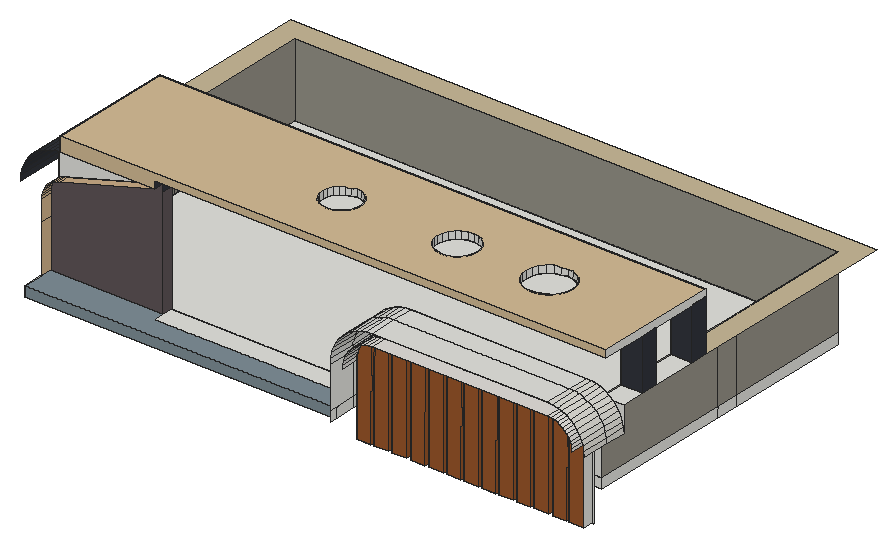
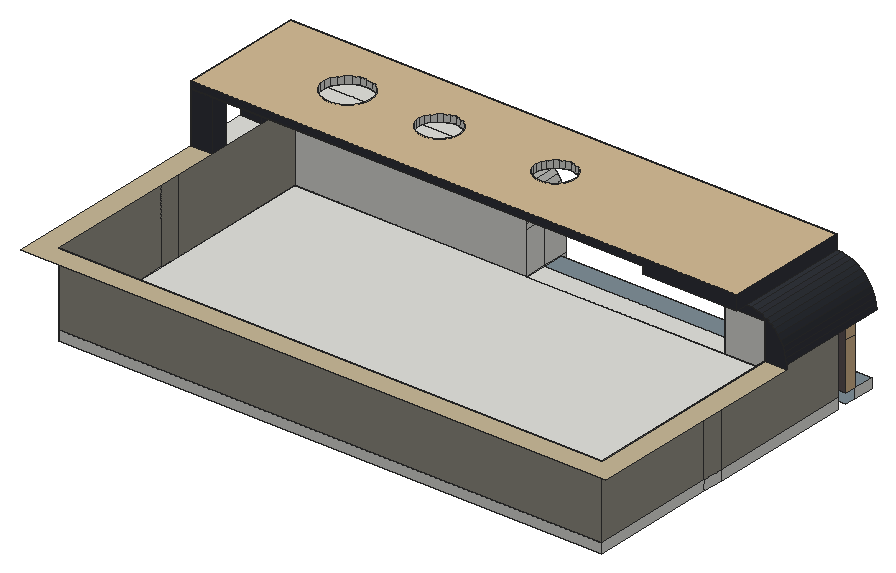
# SketchUp Ruby script. Lengths in inches.
U = 1.inch
M = Sketchup.active_model
def pt(a) = Geom::Point3d.new(a.map { |v| v * U })
def face(e, loops, mat)
  f = e.add_face(loops[0].map { |a| pt(a) })
  loops[1..].each { |l| e.add_face(l.map { |a| pt(a) }).erase! }
  f.material = f.back_material = mat if mat
  f
end
# faces: each face lists its corners as indices into pts; further lists are holes
def faces(e, pts, list, mat = nil) = list.each { |f| face(e, (f[0].is_a?(Array) ? f : [f]).map { |l| l.map { |i| pts[i] } }, mat) }
# xy, xz, yz: faces in a plane at the given z, y or x. An outline is a flat list of corners, or four numbers for a rectangle; further outlines are holes
def ring(l) = l.size == 4 ? [[l[0], l[1]], [l[2], l[1]], [l[2], l[3]], [l[0], l[3]]] : l.each_slice(2).to_a
def flat(e, list, mat, &to3) = list.each { |f| face(e, (f[0].is_a?(Array) ? f : [f]).map { |l| ring(l).map { |u, v| to3.(u, v) } }, mat) }
def xy(e, z, list, mat = nil) = flat(e, list, mat) { |x, y| [x, y, z] }
def xz(e, y, list, mat = nil) = flat(e, list, mat) { |x, z| [x, y, z] }
def yz(e, x, list, mat = nil) = flat(e, list, mat) { |y, z| [x, y, z] }
def lines(e, pts, list) = list.each { |a, b| e.add_line(pt(pts[a]), pt(pts[b])) }
# prism: a flat outline (further loops are holes) pulled along v
def prism(e, loops, v, mat = nil)
  f = face(e, loops, mat); d = Geom::Vector3d.new(v.map { |x| x * U })
  f.pushpull(f.normal.samedirection?(d) ? d.length : -d.length)
end
def box(e, o, s, mat = nil) = prism(e, [[o, [o[0] + s[0], o[1], o[2]], [o[0] + s[0], o[1] + s[1], o[2]], [o[0], o[1] + s[1], o[2]]]], [0, 0, s[2]], mat)
def at(x, y, z, deg = 0) = Geom::Transformation.translation(pt([x, y, z])) * Geom::Transformation.rotation(ORIGIN, Z_AXIS, deg.degrees)
def axes(o, x, y, z) = Geom::Transformation.new([*x, 0, *y, 0, *z, 0, *pt(o).to_a, 1])
def part(name) = M.definitions.add(name)
# library, detail: a bought-in or finely detailed component or shape, given as its bounding box
def library(name, o, s) = part(name).tap { |d| box(d.entities, o, s) }
def detail(e, o, s) = box(e.add_group.entities, o, s)
def put(e, d, t, mat = nil) = e.add_instance(d, t).tap { |i| i.material = mat if mat }
def group(e, t, mat = nil) = e.add_group.tap { |g| g.transformation = t; g.material = mat if mat }.entities
root = M.entities
M.materials.add("[0035_Tan]").color = [210, 180, 140]
M.materials.add("[Asphalt New]").color = [94, 84, 87]
M.materials.add("[Formica Beige]").color = [211, 187, 149]
M.materials.add("[Formica Graystone]1").color = [149, 146, 135]
M.materials.add("[Formica Laminate Dark]").color = [50, 53, 60]
M.materials.add("[Formica Speckled Grey]").color = [127, 142, 150]
M.materials.add("[Quartz Light Brown]").color = [199, 184, 152]
M.materials.add("[Terrazzo Tile Accent]").color = [224, 221, 217]
M.materials.add("[Terrazzo Tile Light]").color = [219, 217, 210]
M.materials.add("[Wood Cherry Original]").color = [152, 86, 42]
xy(root,464.44,[[288.19,14.3125,300.39,22.75],[302.75,14.3125,314.95,22.75],[317.69,14.3125,329.89,22.75],[333.44,14.3125,345.64,22.75],[348.57,14.3125,360.76,22.75],
  [363.5,14.3125,375.7,22.75],[378.19,14.3125,390.39,22.75],[392.75,14.3125,404.95,22.75],[407.44,14.3125,419.64,22.75],[421.94,14.3125,434.14,22.75],
  [436.57,14.3125,448.76,22.75],[452.2,14.3125,464.4,22.75],[466.08,14.3125,478.27,22.75]])
xy(root,479.875,[[112.18,22.75,277.85,40.6875],[17.9375,40.6875,472.4375,162.27],[17.9375,162.27,472.4375,180.28],[17.9375,180.28,472.4375,287.24]])
xy(root,479.875,[[17.9375,5.1875,17.9375,31.75,112.18,31.75,112.18,22.75,277.85,22.75,277.85,5.1875]],"[Formica Speckled Grey]")
xy(root,488.3125,[[112.18,22.75,277.85,40.6875],[17.9375,40.6875,472.4375,287.24]])
xy(root,488.3125,[[17.9375,5.1875,277.85,5.1875,277.85,22.75,112.18,22.75,112.18,31.75,17.9375,31.75]],"[Formica Speckled Grey]")
xy(root,547.97,[[312.85,14.3125,315.18,22.75],[317.69,14.3125,330.02,22.75],[333.44,14.3125,345.77,22.75],[348.57,14.3125,360.9,22.75],[363.5,14.3125,375.83,22.75],
  [378.19,14.3125,390.52,22.75],[392.75,14.3125,405.08,22.75],[407.44,14.3125,419.77,22.75],[421.94,14.3125,434.27,22.75],[436.57,14.3125,448.9,22.75],
  [452.2,14.3125,459.94,22.75]])
xy(root,547.97,[[312.85,0,312.85,14.3125,315.18,14.3125,315.18,22.75,317.69,22.75,317.69,14.3125,330.02,14.3125,330.02,22.75,333.44,22.75,333.44,14.3125,345.77,14.3125,345.77,22.75,348.57,22.75,348.57,14.3125,360.9,14.3125,360.9,22.75,363.5,22.75,363.5,14.3125,375.83,14.3125,375.83,22.75,378.19,22.75,378.19,14.3125,390.52,14.3125,390.52,22.75,392.75,22.75,392.75,14.3125,405.08,14.3125,405.08,22.75,407.44,22.75,407.44,14.3125,419.77,14.3125,419.77,22.75,421.94,22.75,421.94,14.3125,434.27,14.3125,434.27,22.75,436.57,22.75,436.57,14.3125,448.9,14.3125,448.9,22.75,452.2,22.75,452.2,14.3125,459.94,14.3125,459.94,0]],"[Terrazzo Tile Accent]")
xy(root,549.4375,[[472.4375,40.6875,490.375,60.43],[472.4375,60.43,490.375,74.53],[472.4375,74.53,490.375,112.49],[472.4375,112.49,490.375,126.6]])
xy(root,549.4375,[[0,116.75,17.9375,116.75,17.9375,287.24,472.4375,287.24,472.4375,126.6,490.375,126.6,490.375,305.18,0,305.18]],"[Quartz Light Brown]")
xy(root,558.3125,[[312.85,0,459.94,22.75],[312.85,22.75,459.94,40.6875]])
xy(root,579.75,[[17.9375,40.6875,112.18,116.75]])
xy(root,586.1875,[[33.45,22.75,112.18,116.75],[33.45,116.75,112.18,126.6]])
xy(root,592.16,[[[112.18,22.75,490.375,126.6],[402.66,53.0625,407.72,53.73,412.44,55.69,416.49,58.79,419.6,62.85,421.56,67.5625,422.22,72.625,421.56,77.69,419.6,82.41,416.49,86.46,412.44,89.57,407.72,91.52,402.66,92.1875,397.6,91.52,392.88,89.57,388.83,86.46,385.72,82.41,383.76,77.69,383.1,72.625,383.76,67.5625,385.72,62.85,388.83,58.79,392.88,55.69,397.6,53.73],[325.73,55.6875,330.11,56.27,334.2,57.96,337.7,60.65,340.4,64.16,342.09,68.24,342.66,72.625,342.09,77.01,340.4,81.1,337.7,84.6,334.2,87.3,330.11,88.99,325.73,89.5625,321.34,88.99,317.26,87.3,313.75,84.6,311.06,81.1,309.37,77.01,308.79,72.625,309.37,68.24,311.06,64.16,313.75,60.65,317.26,57.96,321.34,56.27],[228.82,56.6875,232.95,57.23,236.79,58.82,240.09,61.36,242.625,64.66,244.22,68.5,244.76,72.625,244.22,76.75,242.625,80.6,240.09,83.9,236.79,86.43,232.95,88.02,228.82,88.5625,224.7,88.02,220.85,86.43,217.55,83.9,215.02,80.6,213.43,76.75,212.89,72.625,213.43,68.5,215.02,64.66,217.55,61.36,220.85,58.82,224.7,57.23]]],"[Formica Beige]")
xy(root,592.3125,[[472.4375,60.43,490.375,74.53],[472.4375,112.49,490.375,126.6]])
xy(root,598.125,[[[33.45,22.75,490.375,126.6],[402.66,53.0625,397.6,53.73,392.88,55.69,388.83,58.79,385.72,62.85,383.76,67.5625,383.1,72.625,383.76,77.69,385.72,82.41,388.83,86.46,392.88,89.57,397.6,91.52,402.66,92.1875,407.72,91.52,412.44,89.57,416.49,86.46,419.6,82.41,421.56,77.69,422.22,72.625,421.56,67.5625,419.6,62.85,416.49,58.79,412.44,55.69,407.72,53.73],[325.73,55.6875,321.34,56.27,317.26,57.96,313.75,60.65,311.06,64.16,309.37,68.24,308.79,72.625,309.37,77.01,311.06,81.1,313.75,84.6,317.26,87.3,321.34,88.99,325.73,89.5625,330.11,88.99,334.2,87.3,337.7,84.6,340.4,81.1,342.09,77.01,342.66,72.625,342.09,68.24,340.4,64.16,337.7,60.65,334.2,57.96,330.11,56.27],[228.82,56.6875,224.7,57.23,220.85,58.82,217.55,61.36,215.02,64.66,213.43,68.5,212.89,72.625,213.43,76.75,215.02,80.6,217.55,83.9,220.85,86.43,224.7,88.02,228.82,88.5625,232.95,88.02,236.79,86.43,240.09,83.9,242.625,80.6,244.22,76.75,244.76,72.625,244.22,68.5,242.625,64.66,240.09,61.36,236.79,58.82,232.95,57.23]]],"[Formica Beige]")
xz(root,5.1875,[[17.9375,479.875,277.85,488.3125]],"[Formica Speckled Grey]")
xz(root,14.3125,[[288.19,464.44,300.39,464.44,300.52,544.67,297.84,542.875,295.41,540.75,293.29,538.32,291.49,535.64,290.07,532.75,289.03,529.69,288.4,526.53,288.19,523.3125],[302.75,464.44,314.95,464.44,315.08,544.67,315.18,547.97,312.85,547.97,309.63,547.76,306.47,547.13,303.41,546.09,302.75,523.3125],[317.69,464.44,329.89,464.44,330.02,544.67,330.02,547.97,317.69,547.97],[333.44,464.44,345.64,464.44,345.77,544.67,345.77,547.97,333.44,547.97],[348.57,464.44,360.76,464.44,360.9,544.67,360.9,547.97,348.57,547.97],
  [363.5,464.44,375.7,464.44,375.83,544.67,375.83,547.97,363.5,547.97],[378.19,464.44,390.39,464.44,390.52,544.67,390.52,547.97,378.19,547.97],[392.75,464.44,404.95,464.44,405.08,544.67,405.08,547.97,392.75,547.97],[407.44,464.44,419.64,464.44,419.77,544.67,419.77,547.97,407.44,547.97],[421.94,464.44,434.14,464.44,434.27,544.67,434.27,547.97,421.94,547.97],
  [436.57,464.44,448.76,464.44,448.9,544.67,448.9,547.97,436.57,547.97],[452.2,464.44,464.4,464.44,464.53,544.67,464.53,547.41,462.57,547.8,459.94,547.97,452.2,547.97],[466.08,464.44,478.27,464.44,478.39,535.8,477.34,537.93,475.88,540.11,474.15,542.09,472.18,543.82,469.99,545.28,467.63,546.44,466.08,546.97]],"[Wood Cherry Original]")
xz(root,22.75,[[288.19,464.44,288.19,523.3125,288.4,526.53,289.03,529.69,290.07,532.75,291.49,535.64,293.29,538.32,295.41,540.75,297.84,542.875,300.52,544.67,300.39,464.44],[302.75,464.44,302.75,523.3125,303.41,546.09,306.47,547.13,309.63,547.76,312.85,547.97,315.18,547.97,315.08,544.67,314.95,464.44],[317.69,464.44,317.69,547.97,330.02,547.97,330.02,544.67,329.89,464.44],[333.44,464.44,333.44,547.97,345.77,547.97,345.77,544.67,345.64,464.44],[348.57,464.44,348.57,547.97,360.9,547.97,360.9,544.67,360.76,464.44],
  [363.5,464.44,363.5,547.97,375.83,547.97,375.83,544.67,375.7,464.44],[378.19,464.44,378.19,547.97,390.52,547.97,390.52,544.67,390.39,464.44],[392.75,464.44,392.75,547.97,405.08,547.97,405.08,544.67,404.95,464.44],[407.44,464.44,407.44,547.97,419.77,547.97,419.77,544.67,419.64,464.44],[421.94,464.44,421.94,547.97,434.27,547.97,434.27,544.67,434.14,464.44],
  [436.57,464.44,436.57,547.97,448.9,547.97,448.9,544.67,448.76,464.44],[452.2,464.44,452.2,547.97,459.94,547.97,462.57,547.8,464.53,547.41,464.53,544.67,464.4,464.44],[466.08,464.44,466.08,546.97,467.63,546.44,469.99,545.28,472.18,543.82,474.15,542.09,475.88,540.11,477.34,537.93,478.39,535.8,478.27,464.44],[478.27,464.44,480.04,464.44,480.04,527.88,479.86,530.5,479.35,533.08,478.51,535.57,478.39,535.8],[478.39,535.8,478.41,544.67,478.41,547.41,476.44,547.8,473.82,547.97,466.08,547.97,466.08,546.97,467.63,546.44,469.99,545.28,472.18,543.82,474.15,542.09,475.88,540.11,477.34,537.93],
  [464.53,547.41,464.53,547.97,459.94,547.97,462.57,547.8]])
xz(root,22.75,[[33.45,586.1875,112.18,586.1875,112.18,592.16,490.375,592.16,490.375,598.125,33.45,598.125]],"[Formica Beige]")
xz(root,22.75,[[300.39,464.44,302.75,464.44,302.75,523.3125,303.41,546.09,300.52,544.67],[314.95,464.44,317.69,464.44,317.69,547.97,315.18,547.97,315.08,544.67],[329.89,464.44,333.44,464.44,333.44,547.97,330.02,547.97,330.02,544.67],[345.64,464.44,348.57,464.44,348.57,547.97,345.77,547.97,345.77,544.67],[360.76,464.44,363.5,464.44,363.5,547.97,360.9,547.97,360.9,544.67],
  [375.7,464.44,378.19,464.44,378.19,547.97,375.83,547.97,375.83,544.67],[390.39,464.44,392.75,464.44,392.75,547.97,390.52,547.97,390.52,544.67],[404.95,464.44,407.44,464.44,407.44,547.97,405.08,547.97,405.08,544.67],[419.64,464.44,421.94,464.44,421.94,547.97,419.77,547.97,419.77,544.67],[434.14,464.44,436.57,464.44,436.57,547.97,434.27,547.97,434.27,544.67],
  [448.76,464.44,452.2,464.44,452.2,547.97,448.9,547.97,448.9,544.67],[464.4,464.44,466.08,464.44,466.08,546.97,465.14,547.29,464.53,547.41,464.53,544.67]],"[Formica Laminate Dark]")
xz(root,31.75,[[17.9375,488.3125,112.18,488.3125,112.18,586.1875,33.29,563.41,31.02,562.96,28.84,562.21,26.77,561.19,24.85,559.91,23.11,558.39,21.59,556.65,20.3,554.73,19.28,552.66,18.54,550.47,18.09,548.21,17.9375,545.9]],"[Asphalt New]")
xz(root,40.6875,[[17.9375,479.875,277.85,488.3125],[277.85,479.875,472.4375,488.3125],[17.9375,488.3125,112.18,579.75],[277.85,488.3125,277.85,523.3125,278.15,527.88,279.04,532.37,280.51,536.71,282.54,540.8125,285.08,544.62,288.1,548.0625,291.54,551.08,295.35,553.625,299.46,555.65,303.79,557.12,308.28,558.01,312.85,558.3125,459.94,558.3125,463.92,558.05,467.82,557.28,471.59,556,472.4375,555.58,472.4375,488.3125],[490.375,527.88,490.375,549.4375,481.42,549.4375,481.46,549.4,484.09,546.41,486.3,543.1,488.06,539.53,489.34,535.76,490.12,531.85],
  [472.4375,549.4375,472.4375,555.58,475.16,554.24,478.47,552.02,481.42,549.4375]])
xz(root,60.43,[[472.4375,549.4375,490.375,592.3125]],"[Formica Laminate Dark]")
xz(root,74.53,[[472.4375,549.4375,490.375,592.3125]],"[Formica Laminate Dark]")
xz(root,112.49,[[472.4375,549.4375,490.375,592.3125]],"[Formica Laminate Dark]")
xz(root,116.75,[[0,549.4375,0,552.73,0.29,557.1,1.14,561.39,2.55,565.54,4.48,569.46,6.91,573.1,9.8,576.39,13.09,579.27,16.73,581.71,17.9375,582.3,17.9375,549.4375],[17.9375,579.75,17.9375,582.3,20.65,583.64,24.8,585.05,29.09,585.9,33.45,586.1875,112.18,586.1875,112.18,579.75]],"[Formica Laminate Dark]")
xz(root,126.6,[[472.4375,592.16,490.375,592.3125]])
xz(root,126.6,[[472.4375,549.4375,490.375,592.16],[33.45,586.1875,33.45,598.125,490.375,598.125,490.375,592.3125,472.4375,592.3125,472.4375,592.16,112.18,592.16,112.18,586.1875]],"[Formica Laminate Dark]")
xz(root,287.24,[[17.9375,479.875,472.4375,488.3125]])
xz(root,287.24,[[17.9375,488.3125,472.4375,549.4375]],"[Formica Graystone]1")
yz(root,17.9375,[[5.1875,479.875,22.75,488.3125],[40.6875,479.875,162.27,488.3125],[162.27,479.875,180.28,488.3125],[180.28,479.875,287.24,488.3125]])
yz(root,17.9375,[[22.75,488.3125,31.75,528.24],[22.75,528.24,31.75,545.9]],"[0035_Tan]")
yz(root,17.9375,[[40.6875,488.3125,162.27,549.4375],[162.27,488.3125,180.28,549.4375],[180.28,488.3125,287.24,549.4375]],"[Formica Graystone]1")
yz(root,17.9375,[[40.6875,549.4375,116.75,579.75]],"[Formica Laminate Dark]")
yz(root,33.45,[[22.75,586.1875,126.6,598.125]],"[Formica Laminate Dark]")
yz(root,112.18,[[31.75,488.3125,40.6875,579.75]],"[Asphalt New]")
yz(root,112.18,[[31.75,579.75,116.75,586.1875],[22.75,586.1875,126.6,592.16]],"[Formica Laminate Dark]")
yz(root,277.85,[[0,479.875,5.1875,488.3125],[5.1875,479.875,22.75,488.3125],[22.75,479.875,40.6875,488.3125],[0,488.3125,22.75,523.3125],[22.75,488.3125,40.6875,523.3125]])
yz(root,288.19,[[14.3125,464.44,22.75,523.3125]])
yz(root,302.75,[[14.3125,464.44,22.75,523.3125]],"[Wood Cherry Original]")
yz(root,317.69,[[14.3125,464.44,22.75,547.97]],"[Wood Cherry Original]")
yz(root,330.02,[[14.3125,544.67,22.75,547.97]],"[Wood Cherry Original]")
yz(root,333.44,[[14.3125,464.44,22.75,547.97]],"[Wood Cherry Original]")
yz(root,345.77,[[14.3125,544.67,22.75,547.97]],"[Wood Cherry Original]")
yz(root,348.57,[[14.3125,464.44,22.75,547.97]],"[Wood Cherry Original]")
yz(root,360.9,[[14.3125,544.67,22.75,547.97]],"[Wood Cherry Original]")
yz(root,363.5,[[14.3125,464.44,22.75,547.97]],"[Wood Cherry Original]")
yz(root,375.83,[[14.3125,544.67,22.75,547.97]],"[Wood Cherry Original]")
yz(root,378.19,[[14.3125,464.44,22.75,547.97]],"[Wood Cherry Original]")
yz(root,390.52,[[14.3125,544.67,22.75,547.97]],"[Wood Cherry Original]")
yz(root,392.75,[[14.3125,464.44,22.75,547.97]],"[Wood Cherry Original]")
yz(root,405.08,[[14.3125,544.67,22.75,547.97]],"[Wood Cherry Original]")
yz(root,407.44,[[14.3125,464.44,22.75,547.97]],"[Wood Cherry Original]")
yz(root,419.77,[[14.3125,544.67,22.75,547.97]],"[Wood Cherry Original]")
yz(root,421.94,[[14.3125,464.44,22.75,547.97]],"[Wood Cherry Original]")
yz(root,434.27,[[14.3125,544.67,22.75,547.97]],"[Wood Cherry Original]")
yz(root,436.57,[[14.3125,464.44,22.75,547.97]],"[Wood Cherry Original]")
yz(root,448.9,[[14.3125,544.67,22.75,547.97]],"[Wood Cherry Original]")
yz(root,452.2,[[14.3125,464.44,22.75,547.97]],"[Wood Cherry Original]")
yz(root,464.53,[[14.3125,544.67,22.75,547.41]],"[Wood Cherry Original]")
yz(root,466.08,[[14.3125,464.44,22.75,546.97]],"[Wood Cherry Original]")
yz(root,472.4375,[[40.6875,479.875,162.27,488.3125],[162.27,479.875,180.28,488.3125],[180.28,479.875,287.24,488.3125]])
yz(root,472.4375,[[40.6875,488.3125,162.27,549.4375],[162.27,488.3125,180.28,549.4375],[180.28,488.3125,287.24,549.4375]],"[Formica Graystone]1")
yz(root,472.4375,[[60.43,549.4375,74.53,592.3125],[112.49,549.4375,126.6,592.3125]],"[Formica Laminate Dark]")
yz(root,490.375,[[22.75,592.16,60.43,592.16,60.43,592.3125,74.53,592.3125,74.53,592.16,112.49,592.16,112.49,592.3125,126.6,592.3125,126.6,598.125,22.75,598.125],[60.43,592.16,74.53,592.3125],[112.49,592.16,126.6,592.3125]])
yz(root,490.375,[[60.43,549.4375,74.53,592.16],[112.49,549.4375,126.6,592.16]],"[Formica Laminate Dark]")
p = [[300.39,22.75,464.44],[300.52,22.75,544.67],[300.52,14.3125,544.67],[300.39,14.3125,464.44],[314.95,22.75,464.44],[315.08,22.75,544.67],
  [315.08,14.3125,544.67],[314.95,14.3125,464.44],[329.89,22.75,464.44],[330.02,22.75,544.67],[330.02,14.3125,544.67],[329.89,14.3125,464.44],
  [345.64,22.75,464.44],[345.77,22.75,544.67],[345.77,14.3125,544.67],[345.64,14.3125,464.44],[360.76,22.75,464.44],[360.9,22.75,544.67],
  [360.9,14.3125,544.67],[360.76,14.3125,464.44],[375.7,22.75,464.44],[375.83,22.75,544.67],[375.83,14.3125,544.67],[375.7,14.3125,464.44],
  [390.39,22.75,464.44],[390.52,22.75,544.67],[390.52,14.3125,544.67],[390.39,14.3125,464.44],[404.95,22.75,464.44],[405.08,22.75,544.67],
  [405.08,14.3125,544.67],[404.95,14.3125,464.44],[419.64,22.75,464.44],[419.77,22.75,544.67],[419.77,14.3125,544.67],[419.64,14.3125,464.44],
  [434.14,22.75,464.44],[434.27,22.75,544.67],[434.27,14.3125,544.67],[434.14,14.3125,464.44],[448.76,22.75,464.44],[448.9,22.75,544.67],
  [448.9,14.3125,544.67],[448.76,14.3125,464.44],[464.4,22.75,464.44],[464.53,22.75,544.67],[464.53,14.3125,544.67],[464.4,14.3125,464.44],
  [478.27,22.75,464.44],[478.39,22.75,535.8],[478.39,14.3125,535.8],[478.27,14.3125,464.44],[278.15,22.75,527.88],[277.85,22.75,523.3125],
  [277.85,0,523.3125],[278.15,0,527.88],[288.19,0,523.3125],[288.19,14.3125,523.3125],[288.4,14.3125,526.53],[288.4,0,526.53],
  [288.19,22.75,523.3125],[288.4,22.75,526.53],[303.41,22.75,546.09],[302.75,22.75,523.3125],[302.75,14.3125,523.3125],[303.41,14.3125,546.09],
  [278.15,40.6875,527.88],[277.85,40.6875,523.3125],[289.03,14.3125,529.69],[289.03,0,529.69],[289.03,22.75,529.69],[279.04,22.75,532.37],
  [279.04,0,532.37],[479.86,22.75,530.5],[480.04,22.75,527.88],[480.04,0,527.88],[479.86,0,530.5],[490.375,22.75,527.88],
  [490.12,22.75,531.85],[490.12,0,531.85],[490.375,0,527.88],[279.04,40.6875,532.37],[490.375,40.6875,527.88],[490.12,40.6875,531.85],
  [290.07,14.3125,532.75],[290.07,0,532.75],[290.07,22.75,532.75],[479.35,22.75,533.08],[479.35,0,533.08],[489.34,22.75,535.76],
  [489.34,0,535.76],[489.34,40.6875,535.76],[280.51,22.75,536.71],[280.51,0,536.71],[280.51,40.6875,536.71],[291.49,14.3125,535.64],
  [291.49,0,535.64],[291.49,22.75,535.64],[478.51,22.75,535.57],[478.51,0,535.57],[293.29,14.3125,538.32],[293.29,0,538.32],
  [477.34,0,537.93],[477.34,14.3125,537.93],[293.29,22.75,538.32],[488.06,22.75,539.53],[488.06,0,539.53],[477.34,22.75,537.93],
  [488.06,40.6875,539.53],[282.54,22.75,540.8125],[282.54,0,540.8125],[282.54,40.6875,540.8125],[475.88,0,540.11],[475.88,14.3125,540.11],
  [475.88,22.75,540.11],[295.41,14.3125,540.75],[295.41,0,540.75],[295.41,22.75,540.75],[486.3,22.75,543.1],[486.3,0,543.1],
  [486.3,40.6875,543.1],[474.15,0,542.09],[474.15,14.3125,542.09],[474.15,22.75,542.09],[297.84,14.3125,542.875],[297.84,0,542.875],
  [297.84,22.75,542.875],[285.08,22.75,544.62],[285.08,0,544.62],[285.08,40.6875,544.62],[472.18,0,543.82],[472.18,14.3125,543.82],
  [472.18,22.75,543.82],[300.52,0,544.67],[484.09,22.75,546.41],[484.09,0,546.41],[484.09,40.6875,546.41],[469.99,0,545.28],
  [469.99,14.3125,545.28],[469.99,22.75,545.28],[288.1,22.75,548.0625],[288.1,0,548.0625],[288.1,40.6875,548.0625],[303.41,0,546.09],
  [315.18,22.75,547.97],[315.18,14.3125,547.97],[467.63,0,546.44],[467.63,14.3125,546.44],[467.63,22.75,546.44],[18.09,22.75,548.21],
  [17.9375,22.75,545.9],[17.9375,31.75,545.9],[18.09,31.75,548.21],[306.47,14.3125,547.13],[306.47,0,547.13],[306.47,22.75,547.13],
  [465.14,22.75,547.29],[466.08,22.75,546.97],[466.08,14.3125,546.97],[465.14,0,547.29],[481.46,22.75,549.4],[481.46,0,549.4],
  [481.46,40.6875,549.4],[309.63,14.3125,547.76],[309.63,0,547.76],[309.63,22.75,547.76],[464.53,22.75,547.41],[462.57,0,547.8],
  [462.57,14.3125,547.8],[464.53,14.3125,547.41],[462.57,22.75,547.8],[312.85,14.3125,547.97],[312.85,0,547.97],[459.94,0,547.97],
  [459.94,14.3125,547.97],[312.85,22.75,547.97],[459.94,22.75,547.97],[291.54,22.75,551.08],[291.54,0,551.08],[291.54,40.6875,551.08],
  [18.54,22.75,550.47],[18.54,31.75,550.47],[478.47,22.75,552.02],[478.47,0,552.02],[481.42,40.6875,549.4375],[478.47,40.6875,552.02],
  [19.28,22.75,552.66],[19.28,31.75,552.66],[295.35,22.75,553.625],[295.35,0,553.625],[295.35,40.6875,553.625],[475.16,22.75,554.24],
  [475.16,0,554.24],[475.16,40.6875,554.24],[0,22.75,552.73],[0.29,22.75,557.1],[0.29,116.75,557.1],[0,116.75,552.73],
  [20.3,22.75,554.73],[20.3,31.75,554.73],[299.46,22.75,555.65],[299.46,0,555.65],[299.46,40.6875,555.65],[471.59,22.75,556],
  [471.59,0,556],[472.4375,40.6875,555.58],[471.59,40.6875,556],[21.59,22.75,556.65],[21.59,31.75,556.65],[303.79,22.75,557.12],
  [303.79,0,557.12],[303.79,40.6875,557.12],[467.82,22.75,557.28],[467.82,0,557.28],[467.82,40.6875,557.28],[23.11,22.75,558.39],
  [23.11,31.75,558.39],[308.28,22.75,558.01],[308.28,0,558.01],[1.14,22.75,561.39],[1.14,116.75,561.39],[308.28,40.6875,558.01],
  [463.92,22.75,558.05],[463.92,0,558.05],[463.92,40.6875,558.05],[312.85,22.75,558.3125],[312.85,0,558.3125],[312.85,40.6875,558.3125],
  [459.94,22.75,558.3125],[459.94,0,558.3125],[459.94,40.6875,558.3125],[24.85,22.75,559.91],[24.85,31.75,559.91],[26.77,22.75,561.19],
  [26.77,31.75,561.19],[28.84,22.75,562.21],[28.84,31.75,562.21],[2.55,22.75,565.54],[2.55,116.75,565.54],[31.02,22.75,562.96],
  [31.02,31.75,562.96],[33.29,22.75,563.41],[33.29,31.75,563.41],[112.18,22.75,586.1875],[112.18,31.75,586.1875],[4.48,22.75,569.46],
  [4.48,116.75,569.46],[6.91,22.75,573.1],[6.91,116.75,573.1],[9.8,22.75,576.39],[9.8,116.75,576.39],[13.09,22.75,579.27],
  [13.09,116.75,579.27],[16.73,22.75,581.71],[16.73,116.75,581.71],[20.65,22.75,583.64],[20.65,116.75,583.64],[17.9375,116.75,582.3],
  [24.8,22.75,585.05],[24.8,116.75,585.05],[29.09,22.75,585.9],[29.09,116.75,585.9],[33.45,22.75,586.1875],[33.45,116.75,586.1875],
  [402.66,53.0625,592.16],[397.6,53.73,592.16],[397.6,53.73,598.125],[402.66,53.0625,598.125],[407.72,53.73,592.16],[407.72,53.73,598.125],
  [392.88,55.69,592.16],[392.88,55.69,598.125],[412.44,55.69,592.16],[412.44,55.69,598.125],[325.73,55.6875,592.16],[321.34,56.27,592.16],
  [321.34,56.27,598.125],[325.73,55.6875,598.125],[330.11,56.27,592.16],[330.11,56.27,598.125],[388.83,58.79,592.16],[388.83,58.79,598.125],
  [416.49,58.79,592.16],[416.49,58.79,598.125],[317.26,57.96,592.16],[317.26,57.96,598.125],[334.2,57.96,592.16],[334.2,57.96,598.125],
  [228.82,56.6875,592.16],[224.7,57.23,592.16],[224.7,57.23,598.125],[228.82,56.6875,598.125],[232.95,57.23,592.16],[232.95,57.23,598.125],
  [220.85,58.82,592.16],[220.85,58.82,598.125],[236.79,58.82,592.16],[236.79,58.82,598.125],[313.75,60.65,592.16],[313.75,60.65,598.125],
  [337.7,60.65,592.16],[337.7,60.65,598.125],[217.55,61.36,592.16],[217.55,61.36,598.125],[240.09,61.36,592.16],[240.09,61.36,598.125],
  [385.72,62.85,592.16],[385.72,62.85,598.125],[419.6,62.85,592.16],[419.6,62.85,598.125],[311.06,64.16,592.16],[311.06,64.16,598.125],
  [340.4,64.16,592.16],[340.4,64.16,598.125],[215.02,64.66,592.16],[215.02,64.66,598.125],[242.625,64.66,592.16],[242.625,64.66,598.125],
  [383.76,67.5625,592.16],[383.76,67.5625,598.125],[421.56,67.5625,592.16],[421.56,67.5625,598.125],[309.37,68.24,592.16],[309.37,68.24,598.125],
  [342.09,68.24,592.16],[342.09,68.24,598.125],[213.43,68.5,592.16],[213.43,68.5,598.125],[244.22,68.5,592.16],[244.22,68.5,598.125],
  [383.1,72.625,592.16],[383.1,72.625,598.125],[422.22,72.625,592.16],[422.22,72.625,598.125],[308.79,72.625,592.16],[308.79,72.625,598.125],
  [342.66,72.625,592.16],[342.66,72.625,598.125],[212.89,72.625,592.16],[212.89,72.625,598.125],[244.76,72.625,592.16],[244.76,72.625,598.125],
  [213.43,76.75,592.16],[213.43,76.75,598.125],[244.22,76.75,592.16],[244.22,76.75,598.125],[309.37,77.01,592.16],[309.37,77.01,598.125],
  [342.09,77.01,592.16],[342.09,77.01,598.125],[383.76,77.69,592.16],[383.76,77.69,598.125],[421.56,77.69,592.16],[421.56,77.69,598.125],
  [215.02,80.6,592.16],[215.02,80.6,598.125],[242.625,80.6,592.16],[242.625,80.6,598.125],[311.06,81.1,592.16],[311.06,81.1,598.125],
  [340.4,81.1,592.16],[340.4,81.1,598.125],[385.72,82.41,592.16],[385.72,82.41,598.125],[419.6,82.41,592.16],[419.6,82.41,598.125],
  [217.55,83.9,592.16],[217.55,83.9,598.125],[240.09,83.9,592.16],[240.09,83.9,598.125],[313.75,84.6,592.16],[313.75,84.6,598.125],
  [337.7,84.6,592.16],[337.7,84.6,598.125],[388.83,86.46,592.16],[388.83,86.46,598.125],[416.49,86.46,592.16],[416.49,86.46,598.125],
  [220.85,86.43,592.16],[220.85,86.43,598.125],[236.79,86.43,592.16],[236.79,86.43,598.125],[317.26,87.3,592.16],[317.26,87.3,598.125],
  [334.2,87.3,592.16],[334.2,87.3,598.125],[224.7,88.02,592.16],[224.7,88.02,598.125],[232.95,88.02,592.16],[232.95,88.02,598.125],
  [392.88,89.57,592.16],[392.88,89.57,598.125],[412.44,89.57,592.16],[412.44,89.57,598.125],[321.34,88.99,592.16],[321.34,88.99,598.125],
  [330.11,88.99,592.16],[330.11,88.99,598.125],[228.82,88.5625,592.16],[228.82,88.5625,598.125],[325.73,89.5625,592.16],[325.73,89.5625,598.125],
  [397.6,91.52,592.16],[397.6,91.52,598.125],[407.72,91.52,592.16],[407.72,91.52,598.125],[402.66,92.1875,592.16],[402.66,92.1875,598.125]]
faces(root,p,[[0,1,2,3],[4,5,6,7],[8,9,10,11],[12,13,14,15],[16,17,18,19],[20,21,22,23],[24,25,26,27],[28,29,30,31],
  [32,33,34,35],[36,37,38,39],[40,41,42,43],[44,45,46,47],[62,63,64,65],[5,144,145,6]],"[Wood Cherry Original]")
faces(root,p,[[48,49,50,51],[52,53,54,55],[60,61,58,57],[53,52,66,67],[61,70,68,58],[71,52,55,72],[52,71,81,66],[70,86,84,68],
  [92,71,72,93],[71,92,94,81],[86,97,95,84],[97,104,100,95],[107,49,50,103],[109,92,93,110],[92,109,111,94],[114,107,103,113],
  [104,117,115,100],[123,114,113,122],[117,126,124,115],[127,109,110,128],[109,127,129,111],[132,123,122,131],[126,1,2,124],[139,132,131,138],
  [140,127,128,141],[127,140,142,129],[148,139,138,147],[62,155,153,65],[157,148,147,158],[155,165,163,153],[170,166,169,168],[165,175,171,163],
  [176,170,168,174],[177,140,141,178],[140,177,179,142],[188,177,178,189],[177,188,190,179],[200,188,189,201],[188,200,202,190],[209,200,201,210],
  [200,209,211,202],[217,209,210,218],[209,217,221,211],[225,217,218,226],[217,225,227,221],[264,265,266,267],[268,264,267,269],[265,270,271,266],
  [272,268,269,273],[274,275,276,277],[278,274,277,279],[270,280,281,271],[282,272,273,283],[275,284,285,276],[286,278,279,287],[288,289,290,291],
  [292,288,291,293],[289,294,295,290],[296,292,293,297],[284,298,299,285],[300,286,287,301],[294,302,303,295],[304,296,297,305],[280,306,307,281],
  [308,282,283,309],[298,310,311,299],[312,300,301,313],[302,314,315,303],[316,304,305,317],[306,318,319,307],[320,308,309,321],[310,322,323,311],
  [324,312,313,325],[314,326,327,315],[328,316,317,329],[318,330,331,319],[332,320,321,333],[322,334,335,323],[336,324,325,337],[326,338,339,327],
  [340,328,329,341],[338,342,343,339],[344,340,341,345],[334,346,347,335],[348,336,337,349],[330,350,351,331],[352,332,333,353],[342,354,355,343],
  [356,344,345,357],[346,358,359,347],[360,348,349,361],[350,362,363,351],[364,352,353,365],[354,366,367,355],[368,356,357,369],[358,370,371,359],
  [372,360,361,373],[362,374,375,363],[376,364,365,377],[366,378,379,367],[380,368,369,381],[370,382,383,371],[384,372,373,385],[378,386,387,379],
  [388,380,381,389],[374,390,391,375],[392,376,377,393],[382,394,395,383],[396,384,385,397],[386,398,399,387],[398,388,389,399],[394,400,401,395],
  [400,396,397,401],[390,402,403,391],[404,392,393,405],[402,406,407,403],[406,404,405,407]])
faces(root,p,[[56,57,58,59],[59,58,68,69],[73,74,75,76],[69,68,84,85],[87,73,76,88],[85,84,95,96],[98,87,88,99],[96,95,100,101],
  [49,98,99,102,103,50],[112,113,103,102],[101,100,115,116],[121,122,113,112],[116,115,124,125],[130,131,122,121],[125,124,2,133],[137,138,131,130],
  [1,62,65,143,133,2],[146,147,138,137],[143,65,153,154],[156,157,158,147,146,159],[154,153,163,164],[166,156,159,167,168,169],[164,163,171,172],[173,174,168,167]],"[Terrazzo Tile Accent]")
faces(root,p,[[77,78,79,80],[78,77,82,83],[78,89,90,79],[89,78,83,91],[89,105,106,90],[105,89,91,108],[105,118,119,106],[118,105,108,120],
  [118,134,135,119],[134,118,120,136],[134,160,161,135],[160,134,136,162],[160,182,183,161],[182,160,162,184,185],[182,191,192,183],[191,182,185,193],
  [191,203,204,192],[203,191,193,205,206],[203,212,213,204],[212,203,206,214],[212,222,223,213],[222,212,214,224],[222,228,229,223],[228,222,224,230]],"[Terrazzo Tile Light]")
faces(root,p,[[149,150,151,152],[180,149,152,181],[186,180,181,187],[198,186,187,199],[207,198,199,208],[215,207,208,216],[231,215,216,232],[233,231,232,234],
  [235,233,234,236],[239,235,236,240],[241,239,240,242],[243,241,242,244]],"[0035_Tan]")
faces(root,p,[[194,195,196,197],[195,219,220,196],[219,237,238,220],[237,245,246,238],[245,247,248,246],[247,249,250,248],[249,251,252,250],[251,253,254,252],
  [253,255,256,257,254],[255,258,259,256],[258,260,261,259],[260,262,263,261]],"[Formica Laminate Dark]")
